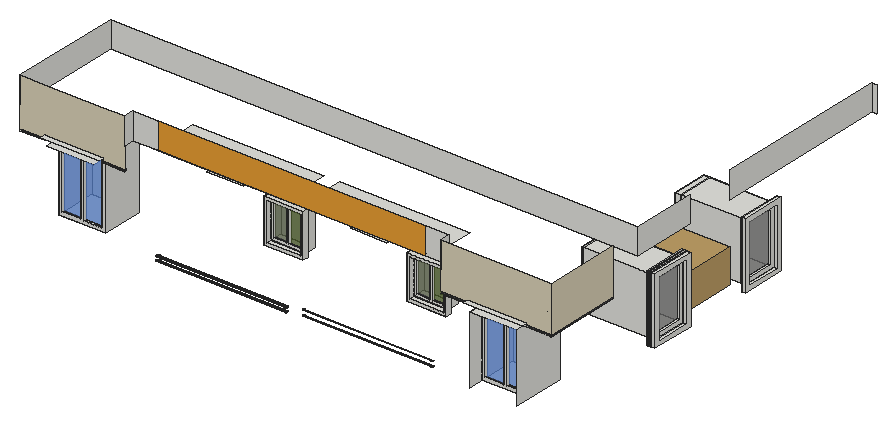
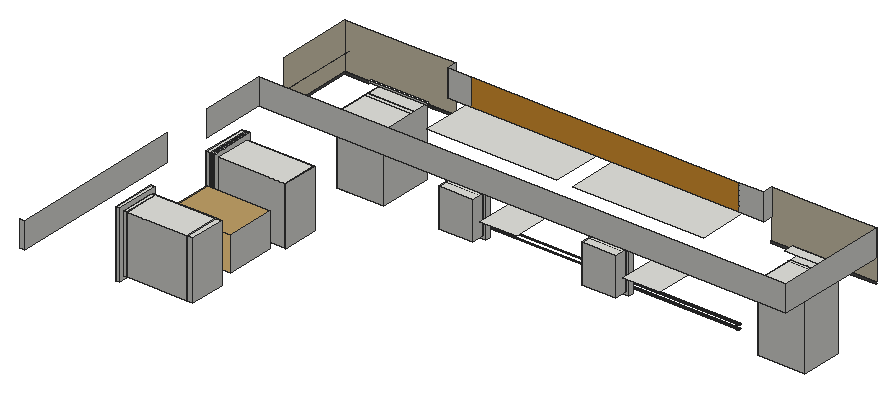
# SketchUp Ruby script. Lengths in inches.
U = 1.inch
M = Sketchup.active_model
def pt(a) = Geom::Point3d.new(a.map { |v| v * U })
def face(e, loops, mat)
  f = e.add_face(loops[0].map { |a| pt(a) })
  loops[1..].each { |l| e.add_face(l.map { |a| pt(a) }).erase! }
  f.material = f.back_material = mat if mat
  f
end
# faces: each face lists its corners as indices into pts; further lists are holes
def faces(e, pts, list, mat = nil) = list.each { |f| face(e, (f[0].is_a?(Array) ? f : [f]).map { |l| l.map { |i| pts[i] } }, mat) }
# xy, xz, yz: faces in a plane at the given z, y or x. An outline is a flat list of corners, or four numbers for a rectangle; further outlines are holes
def ring(l) = l.size == 4 ? [[l[0], l[1]], [l[2], l[1]], [l[2], l[3]], [l[0], l[3]]] : l.each_slice(2).to_a
def flat(e, list, mat, &to3) = list.each { |f| face(e, (f[0].is_a?(Array) ? f : [f]).map { |l| ring(l).map { |u, v| to3.(u, v) } }, mat) }
def xy(e, z, list, mat = nil) = flat(e, list, mat) { |x, y| [x, y, z] }
def xz(e, y, list, mat = nil) = flat(e, list, mat) { |x, z| [x, y, z] }
def yz(e, x, list, mat = nil) = flat(e, list, mat) { |y, z| [x, y, z] }
def lines(e, pts, list) = list.each { |a, b| e.add_line(pt(pts[a]), pt(pts[b])) }
# prism: a flat outline (further loops are holes) pulled along v
def prism(e, loops, v, mat = nil)
  f = face(e, loops, mat); d = Geom::Vector3d.new(v.map { |x| x * U })
  f.pushpull(f.normal.samedirection?(d) ? d.length : -d.length)
end
def box(e, o, s, mat = nil) = prism(e, [[o, [o[0] + s[0], o[1], o[2]], [o[0] + s[0], o[1] + s[1], o[2]], [o[0], o[1] + s[1], o[2]]]], [0, 0, s[2]], mat)
def at(x, y, z, deg = 0) = Geom::Transformation.translation(pt([x, y, z])) * Geom::Transformation.rotation(ORIGIN, Z_AXIS, deg.degrees)
def axes(o, x, y, z) = Geom::Transformation.new([*x, 0, *y, 0, *z, 0, *pt(o).to_a, 1])
def part(name) = M.definitions.add(name)
# library, detail: a bought-in or finely detailed component or shape, given as its bounding box
def library(name, o, s) = part(name).tap { |d| box(d.entities, o, s) }
def detail(e, o, s) = box(e.add_group.entities, o, s)
def put(e, d, t, mat = nil) = e.add_instance(d, t).tap { |i| i.material = mat if mat }
def group(e, t, mat = nil) = e.add_group.tap { |g| g.transformation = t; g.material = mat if mat }.entities
root = M.entities
M.materials.add("Generic").color = [191, 159, 103]
M.materials.add("Generic\#1").color = [233, 159, 52]
M.materials.add("Generic\#3").color = [218, 209, 183]
M.materials.add("[Color M06]").color = [86, 86, 86]
M.materials.add("[Translucent Glass Blue]").color = [100, 149, 237]
M.materials["[Translucent Glass Blue]"].alpha = 0.5
M.materials.add("[Translucent Glass Dark Green]").color = [62, 91, 5]
M.materials["[Translucent Glass Dark Green]"].alpha = 0.5
M.materials.add("[Translucent Glass Gray]").color = [128, 128, 128]
M.materials["[Translucent Glass Gray]"].alpha = 0.5
c1 = part("Group\#1")
xy(c1.entities,0,[[0,0,71.4375,6]])
xy(c1.entities,5.26,[[5.26,0,33.09,3],[38.35,0,66.18,3]])
xy(c1.entities,97.49,[[5.26,0,33.09,3],[38.35,0,66.18,3]])
xy(c1.entities,102.75,[[0,0,71.4375,6]])
xz(c1.entities,0,[[[0,0,71.4375,102.75],[38.35,5.26,66.18,97.49],[5.26,5.26,33.09,97.49]]])
xz(c1.entities,3,[[5.26,5.26,33.09,97.49],[38.35,5.26,66.18,97.49]],"[Translucent Glass Blue]")
xz(c1.entities,6,[[0,0,71.4375,102.75]],"[Translucent Glass Blue]")
yz(c1.entities,0,[[0,0,6,102.75]])
yz(c1.entities,5.26,[[0,5.26,3,97.49]])
yz(c1.entities,33.09,[[0,5.26,3,97.49]])
yz(c1.entities,38.35,[[0,5.26,3,97.49]])
yz(c1.entities,66.18,[[0,5.26,3,97.49]])
yz(c1.entities,71.4375,[[0,0,6,102.75]])
c2 = part("Group\#7")
xy(c2.entities,0,[[0,0,6,54.3125]])
xy(c2.entities,5.9,[[3,5.9,6,48.41]])
xy(c2.entities,81.98,[[3,5.9,6,48.41]])
xy(c2.entities,87.88,[[0,0,6,54.3125]])
xz(c2.entities,0,[[0,0,6,87.88]])
xz(c2.entities,5.9,[[3,5.9,6,81.98]])
xz(c2.entities,48.41,[[3,5.9,6,81.98]])
xz(c2.entities,54.3125,[[0,0,6,87.88]])
yz(c2.entities,0,[[0,0,54.3125,87.88]],"[Translucent Glass Gray]")
yz(c2.entities,3,[[5.9,5.9,48.41,81.98]],"[Translucent Glass Gray]")
yz(c2.entities,6,[[[0,0,54.3125,87.88],[5.9,5.9,48.41,81.98]]])
c3 = part("Group\#3")
xy(c3.entities,0,[[0,0,51.8125,6]])
xy(c3.entities,4.04,[[4.04,0,23.89,3],[27.93,0,47.77,3]])
xy(c3.entities,53.71,[[4.04,0,23.89,3],[27.93,0,47.77,3]])
xy(c3.entities,57.75,[[0,0,51.8125,6]])
xz(c3.entities,0,[[[0,0,51.8125,57.75],[4.04,4.04,23.89,53.71],[27.93,4.04,47.77,53.71]]])
xz(c3.entities,3,[[4.04,4.04,23.89,53.71],[27.93,4.04,47.77,53.71]],"[Translucent Glass Dark Green]")
xz(c3.entities,6,[[0,0,51.8125,57.75]],"[Translucent Glass Gray]")
yz(c3.entities,0,[[0,0,6,57.75]])
yz(c3.entities,4.04,[[0,4.04,3,53.71]])
yz(c3.entities,23.89,[[0,4.04,3,53.71]])
yz(c3.entities,27.93,[[0,4.04,3,53.71]])
yz(c3.entities,47.77,[[0,4.04,3,53.71]])
yz(c3.entities,51.8125,[[0,0,6,57.75]])
xy(root,699.45,[[50,83.8125,121.4375,146.5625]])
xy(root,700.06,[[691.41,83.8125,762.85,142.1875]])
xy(root,710.22,[[802.875,257.24,804.9375,324.36],[804.9375,257.24,807,324.36],[807,257.24,809.375,324.36],[809.375,257.24,815.3125,324.36],[809.375,428.47,815.3125,495.59]])
xy(root,716.625,[[699,263.64,701.375,317.96],[701.375,263.64,802.875,317.96],[802.875,263.64,804.9375,317.96],[804.9375,263.64,807,317.96],[807,263.64,809.375,317.96],
  [809.375,263.64,815.3125,317.96],[703.4375,434.88,712.375,489.19],[712.375,434.88,802.875,489.19],[802.875,434.88,809.375,489.19],[809.375,434.88,815.3125,489.19]])
xy(root,719.55,[[307.73,150.125,367.625,158.75],[524.6,150.125,584.5,158.75]])
xy(root,722.9375,[[706.68,338.625,802.875,413.6875]],"Generic")
xy(root,723.59,[[311.77,150.125,363.58,158.75],[528.64,150.125,580.46,158.75],[311.77,158.75,363.58,177.1875],[528.64,158.75,580.46,177.1875]])
xy(root,774.4375,[[706.68,338.625,802.875,413.6875]],"Generic")
xy(root,781.34,[[311.77,150.125,363.58,158.75],[528.64,150.125,580.46,158.75],[311.77,158.75,363.58,177.1875],[528.64,158.75,580.46,177.1875]])
xy(root,782.3125,[[215.38,158.75,271.07,214.75],[432.26,158.75,487.94,214.75]])
xy(root,785.38,[[307.73,150.125,367.625,158.75],[524.6,150.125,584.5,158.75]])
xy(root,802.2,[[50,60.5625,121.4375,83.8125],[50,83.8125,121.4375,146.5625]])
xy(root,802.81,[[691.41,60.5625,762.85,142.1875]])
xy(root,803.75,[[4.1875,68.5,41.1,69.9375],[130.34,68.5,162.33,69.9375]])
xy(root,804.5,[[699,263.64,701.375,317.96],[701.375,263.64,802.875,317.96],[802.875,263.64,804.9375,317.96],[804.9375,263.64,807,317.96],[807,263.64,809.375,317.96],
  [809.375,263.64,815.3125,317.96],[703.4375,434.88,712.375,489.19],[712.375,434.88,802.875,489.19],[802.875,434.88,809.375,489.19],[809.375,434.88,815.3125,489.19]])
xy(root,806.5,[[641.55,68.5,682.51,69.9375],[771.75,68.5,802.875,69.9375],[802.875,68.5,809.375,69.9375],[807.9375,69.9375,809.375,185.01]])
xy(root,806.75,[[4.1875,68.5,41.1,69.9375],[130.34,68.5,162.33,69.9375]])
xy(root,809.5,[[641.55,68.5,682.51,69.9375],[771.75,68.5,809.375,69.9375],[807.9375,69.9375,809.375,185.01]])
xy(root,810.91,[[802.875,257.24,804.9375,324.36],[804.9375,257.24,807,324.36],[807,257.24,809.375,324.36],[809.375,257.24,815.3125,324.36],[809.375,428.47,815.3125,495.59]])
xy(root,811.1,[[41.1,60.5625,130.34,68.5],[41.1,68.5,130.34,83.8125]])
xy(root,811.71,[[682.51,60.5625,771.75,68.5]])
xy(root,839.25,[[193.83,83.8125,391.53,158.75],[415.53,83.8125,613.23,158.75]])
xz(root,68.5,[[129.35,803.75,130.34,806.75],[682.51,806.5,771.75,809.5]])
xz(root,68.5,[[4.1875,806.75,41.1,806.75,41.1,811.1,130.34,811.1,130.34,806.75,162.33,806.75,162.33,879,129.35,879,129.35,878.57,40.11,878.57,40.11,879,4.1875,879],[641.55,809.5,682.51,809.5,682.51,811.71,771.75,811.71,771.75,809.5,809.375,809.5,809.375,879,771.75,879,771.75,878.32,682.51,878.32,682.51,879,641.55,879]],"Generic\#3")
xz(root,69.9375,[[4.1875,803.75,41.1,806.75],[130.34,803.75,162.33,806.75],[641.55,806.5,682.51,809.5],[771.75,806.5,807.9375,809.5]],"[Color M06]")
xz(root,83.8125,[[162.33,839.25,200.02,879],[607.05,839.25,641.55,879]])
xz(root,83.8125,[[200.02,839.25,607.05,879]],"Generic\#1")
xz(root,142.1875,[[691.41,700.06,762.85,802.81]])
xz(root,146.5625,[[50,699.45,121.4375,802.2]])
xz(root,150.125,[[[307.73,719.55,367.625,785.38],[311.77,723.59,363.58,781.34]],[[524.6,719.55,584.5,785.38],[528.64,723.59,580.46,781.34]]])
xz(root,158.75,[[[307.73,719.55,367.625,785.38],[311.77,723.59,363.58,781.34]],[[524.6,719.55,584.5,785.38],[528.64,723.59,580.46,781.34]]])
xz(root,177.1875,[[311.77,723.59,363.58,781.34],[528.64,723.59,580.46,781.34]])
xz(root,185.01,[[807.9375,806.5,809.375,809.5]])
xz(root,239.73,[[4.1875,839.25,802.875,879]])
xz(root,257.24,[[802.875,710.22,804.9375,810.91],[804.9375,710.22,807,810.91],[807,710.22,809.375,810.91],[809.375,710.22,815.3125,810.91]])
xz(root,263.64,[[699,716.625,701.375,804.5],[701.375,716.625,802.875,804.5],[802.875,716.625,804.9375,804.5],[804.9375,716.625,807,804.5],[807,716.625,809.375,804.5],
  [809.375,716.625,815.3125,804.5]])
xz(root,317.96,[[699,716.625,701.375,804.5],[701.375,716.625,802.875,804.5],[802.875,716.625,804.9375,804.5],[804.9375,716.625,807,804.5],[807,716.625,809.375,804.5],
  [809.375,716.625,815.3125,804.5]])
xz(root,324.36,[[802.875,710.22,804.9375,810.91],[804.9375,710.22,807,810.91],[807,710.22,809.375,810.91],[809.375,710.22,815.3125,810.91]])
xz(root,428.47,[[809.375,710.22,815.3125,810.91]])
xz(root,434.88,[[703.4375,716.625,712.375,804.5],[712.375,716.625,802.875,804.5],[802.875,716.625,809.375,804.5],[809.375,716.625,815.3125,804.5]])
xz(root,489.19,[[703.4375,716.625,712.375,804.5],[712.375,716.625,802.875,804.5],[802.875,716.625,809.375,804.5],[809.375,716.625,815.3125,804.5]])
xz(root,495.59,[[809.375,710.22,815.3125,810.91]])
xz(root,683.8125,[[802.875,839.25,809.375,879]])
yz(root,4.1875,[[68.5,839.25,239.73,879]])
yz(root,50,[[83.8125,699.45,146.5625,802.2]])
yz(root,121.4375,[[83.8125,699.45,146.5625,802.2]])
yz(root,130.34,[[68.5,803.75,69.9375,806.75]])
yz(root,162.33,[[68.5,839.25,83.8125,879]])
yz(root,307.73,[[150.125,719.55,158.75,785.38]])
yz(root,311.77,[[150.125,723.59,158.75,781.34],[158.75,723.59,177.1875,781.34]])
yz(root,363.58,[[150.125,723.59,158.75,781.34],[158.75,723.59,177.1875,781.34]])
yz(root,367.625,[[150.125,719.55,158.75,785.38]])
yz(root,524.6,[[150.125,719.55,158.75,785.38]])
yz(root,528.64,[[150.125,723.59,158.75,781.34],[158.75,723.59,177.1875,781.34]])
yz(root,580.46,[[150.125,723.59,158.75,781.34],[158.75,723.59,177.1875,781.34]])
yz(root,584.5,[[150.125,719.55,158.75,785.38]])
yz(root,641.55,[[68.5,839.25,83.8125,879]])
yz(root,682.51,[[68.5,806.5,69.9375,809.5]])
yz(root,691.41,[[60.5625,700.06,142.1875,802.81]])
yz(root,699,[[263.64,716.625,317.96,804.5]])
yz(root,701.375,[[263.64,716.625,317.96,804.5]])
yz(root,703.4375,[[434.88,716.625,489.19,804.5]])
yz(root,706.68,[[338.625,722.9375,413.6875,774.4375]])
yz(root,712.375,[[434.88,716.625,489.19,804.5]])
yz(root,762.85,[[60.5625,700.06,142.1875,802.81]])
yz(root,771.75,[[68.5,806.5,69.9375,809.5]])
yz(root,802.875,[[[257.24,710.22,324.36,810.91],[263.64,716.625,317.96,804.5]],[239.73,839.25,338.625,879],[413.6875,839.25,683.8125,879]])
yz(root,802.875,[[338.625,722.9375,413.6875,774.4375]],"Generic")
yz(root,804.9375,[[[257.24,710.22,324.36,810.91],[263.64,716.625,317.96,804.5]]])
yz(root,807,[[[257.24,710.22,324.36,810.91],[263.64,716.625,317.96,804.5]]])
yz(root,807.9375,[[69.9375,806.5,185.01,809.5]],"[Color M06]")
yz(root,809.375,[[[257.24,710.22,324.36,810.91],[263.64,716.625,317.96,804.5]],[[428.47,710.22,495.59,810.91],[434.88,716.625,489.19,804.5]]])
yz(root,809.375,[[68.5,809.5,185.01,879]],"Generic\#3")
yz(root,815.3125,[[[257.24,710.22,324.36,810.91],[263.64,716.625,317.96,804.5]],[[428.47,710.22,495.59,810.91],[434.88,716.625,489.19,804.5]]])
p = [[193.83,89.44,683.74],[193.83,89.73,683.625],[391.53,89.73,683.625],[391.53,89.44,683.74],[193.83,90.04,683.58],[391.53,90.04,683.58],
  [193.83,90.35,683.625],[391.53,90.35,683.625],[193.83,90.63,683.74],[391.53,90.63,683.74],[193.83,89.2,683.93],[391.53,89.2,683.93],
  [193.83,90.88,683.93],[391.53,90.88,683.93],[193.83,89.01,684.18],[391.53,89.01,684.18],[193.83,91.07,684.18],[391.53,91.07,684.18],
  [193.83,88.89,684.46],[391.53,88.89,684.46],[193.83,91.18,684.46],[391.53,91.18,684.46],[193.83,88.85,684.77],[391.53,88.85,684.77],
  [193.83,91.23,684.77],[391.53,91.23,684.77],[193.83,88.89,685.08],[391.53,88.89,685.08],[193.83,91.18,685.08],[391.53,91.18,685.08],
  [193.83,89.01,685.36],[391.53,89.01,685.36],[193.83,91.07,685.36],[391.53,91.07,685.36],[193.83,89.2,685.61],[391.53,89.2,685.61],
  [193.83,90.88,685.61],[391.53,90.88,685.61],[193.83,89.44,685.8],[391.53,89.44,685.8],[193.83,90.63,685.8],[391.53,90.63,685.8],
  [193.83,89.73,685.92],[391.53,89.73,685.92],[193.83,90.35,685.92],[391.53,90.35,685.92],[193.83,90.04,685.96],[391.53,90.04,685.96],
  [415.53,88.8125,688.125],[415.53,88.93,688.04],[613.23,88.93,688.04],[613.23,88.8125,688.125],[415.53,89.0625,687.98],[613.23,89.0625,687.98],
  [415.53,89.21,687.96],[613.23,89.21,687.96],[415.53,89.36,687.98],[613.23,89.36,687.98],[415.53,89.49,688.04],[613.23,89.49,688.04],
  [415.53,89.61,688.125],[613.23,89.61,688.125],[415.53,88.72,688.24],[613.23,88.72,688.24],[415.53,89.7,688.24],[613.23,89.7,688.24],
  [415.53,88.67,688.38],[613.23,88.67,688.38],[415.53,89.75,688.38],[613.23,89.75,688.38],[415.53,88.65,688.52],[613.23,88.65,688.52],
  [415.53,89.77,688.52],[613.23,89.77,688.52],[415.53,88.67,688.67],[613.23,88.67,688.67],[415.53,89.75,688.67],[613.23,89.75,688.67],
  [415.53,88.72,688.81],[613.23,88.72,688.81],[415.53,89.7,688.81],[613.23,89.7,688.81],[415.53,88.8125,688.92],[613.23,88.8125,688.92],
  [415.53,89.61,688.92],[613.23,89.61,688.92],[415.53,88.93,689.01],[613.23,88.93,689.01],[415.53,89.49,689.01],[613.23,89.49,689.01],
  [415.53,89.0625,689.07],[613.23,89.0625,689.07],[415.53,89.36,689.07],[613.23,89.36,689.07],[415.53,89.21,689.09],[613.23,89.21,689.09],
  [193.83,89.73,690.1875],[193.83,90.04,690.15],[391.53,90.04,690.15],[391.53,89.73,690.1875],[193.83,90.35,690.1875],[391.53,90.35,690.1875],
  [193.83,89.44,690.31],[391.53,89.44,690.31],[193.83,90.63,690.31],[391.53,90.63,690.31],[193.83,89.2,690.49],[391.53,89.2,690.49],
  [193.83,90.88,690.49],[391.53,90.88,690.49],[193.83,89.01,690.74],[391.53,89.01,690.74],[193.83,91.07,690.74],[391.53,91.07,690.74],
  [193.83,88.89,691.03],[391.53,88.89,691.03],[193.83,91.18,691.03],[391.53,91.18,691.03],[193.83,88.85,691.33],[391.53,88.85,691.33],
  [193.83,91.23,691.33],[391.53,91.23,691.33],[193.83,88.89,691.64],[391.53,88.89,691.64],[193.83,91.18,691.64],[391.53,91.18,691.64],
  [193.83,89.01,691.93],[391.53,89.01,691.93],[193.83,91.07,691.93],[391.53,91.07,691.93],[193.83,89.2,692.17],[391.53,89.2,692.17],
  [193.83,90.88,692.17],[391.53,90.88,692.17],[193.83,89.44,692.36],[391.53,89.44,692.36],[193.83,90.63,692.36],[391.53,90.63,692.36],
  [193.83,89.73,692.48],[391.53,89.73,692.48],[193.83,90.35,692.48],[391.53,90.35,692.48],[193.83,90.04,692.52],[391.53,90.04,692.52],
  [415.53,88.93,695.47],[415.53,89.0625,695.42],[613.23,89.0625,695.42],[613.23,88.93,695.47],[415.53,89.21,695.4],[613.23,89.21,695.4],
  [415.53,89.36,695.42],[613.23,89.36,695.42],[415.53,89.49,695.47],[613.23,89.49,695.47],[415.53,88.8125,695.5625],[613.23,88.8125,695.5625],
  [415.53,89.61,695.5625],[613.23,89.61,695.5625],[415.53,88.72,695.68],[613.23,88.72,695.68],[415.53,89.7,695.68],[613.23,89.7,695.68],
  [415.53,88.67,695.82],[613.23,88.67,695.82],[415.53,89.75,695.82],[613.23,89.75,695.82],[415.53,88.65,695.96],[613.23,88.65,695.96],
  [415.53,89.77,695.96],[613.23,89.77,695.96],[415.53,88.67,696.11],[613.23,88.67,696.11],[415.53,89.75,696.11],[613.23,89.75,696.11],
  [415.53,88.72,696.24],[613.23,88.72,696.24],[415.53,89.7,696.24],[613.23,89.7,696.24],[415.53,88.8125,696.36],[613.23,88.8125,696.36],
  [415.53,89.61,696.36],[613.23,89.61,696.36],[415.53,88.93,696.45],[613.23,88.93,696.45],[415.53,89.0625,696.51],[613.23,89.0625,696.51],
  [415.53,89.49,696.45],[415.53,89.36,696.51],[613.23,89.36,696.51],[613.23,89.49,696.45],[415.53,89.21,696.52],[613.23,89.21,696.52],
  [802.875,68.5,839.25],[802.875,185.01,839.25],[415.53,89.21,695.9],[613.23,89.21,695.9],[415.53,89.21,688.46],[613.23,89.21,688.46],
  [193.83,90.04,684.33],[391.53,90.04,684.33],[193.83,90.04,691.08],[391.53,90.04,691.08]]
faces(root,p,[[0,1,2,3],[1,4,5,2],[4,6,7,5],[6,8,9,7],[10,0,3,11],[8,12,13,9],[14,10,11,15],[12,16,17,13],
  [18,14,15,19],[16,20,21,17],[22,18,19,23],[20,24,25,21],[26,22,23,27],[24,28,29,25],[30,26,27,31],[28,32,33,29],
  [34,30,31,35],[32,36,37,33],[38,34,35,39],[36,40,41,37],[42,38,39,43],[40,44,45,41],[46,42,43,47],[44,46,47,45],
  [48,49,50,51],[49,52,53,50],[52,54,55,53],[54,56,57,55],[56,58,59,57],[58,60,61,59],[62,48,51,63],[60,64,65,61],
  [66,62,63,67],[64,68,69,65],[70,66,67,71],[68,72,73,69],[74,70,71,75],[72,76,77,73],[78,74,75,79],[76,80,81,77],
  [82,78,79,83],[80,84,85,81],[86,82,83,87],[84,88,89,85],[90,86,87,91],[88,92,93,89],[94,90,91,95],[92,94,95,93],
  [96,97,98,99],[97,100,101,98],[102,96,99,103],[100,104,105,101],[106,102,103,107],[104,108,109,105],[110,106,107,111],[108,112,113,109],
  [114,110,111,115],[112,116,117,113],[118,114,115,119],[116,120,121,117],[122,118,119,123],[120,124,125,121],[126,122,123,127],[124,128,129,125],
  [130,126,127,131],[128,132,133,129],[134,130,131,135],[132,136,137,133],[138,134,135,139],[136,140,141,137],[142,138,139,143],[140,142,143,141],
  [144,145,146,147],[145,148,149,146],[148,150,151,149],[150,152,153,151],[154,144,147,155],[152,156,157,153],[158,154,155,159],[156,160,161,157],
  [162,158,159,163],[160,164,165,161],[166,162,163,167],[164,168,169,165],[170,166,167,171],[168,172,173,169],[174,170,171,175],[172,176,177,173],
  [178,174,175,179],[176,180,181,177],[182,178,179,183],[184,182,183,185],[186,187,188,189],[180,186,189,181],[190,184,185,191],[187,190,191,188]])
lines(root,p,[[192,193],[194,195],[196,197],[198,199],[200,201]])
put(root,c1,at(50,83.8125,699.45))
put(root,c1,at(691.41,83.8125,700.06))
put(root,c2,at(803.375,434.88,716.625))
put(root,c2,at(803.375,263.64,716.625))
put(root,c3,at(311.77,158.75,723.59))
put(root,c3,at(528.64,158.75,723.59))
